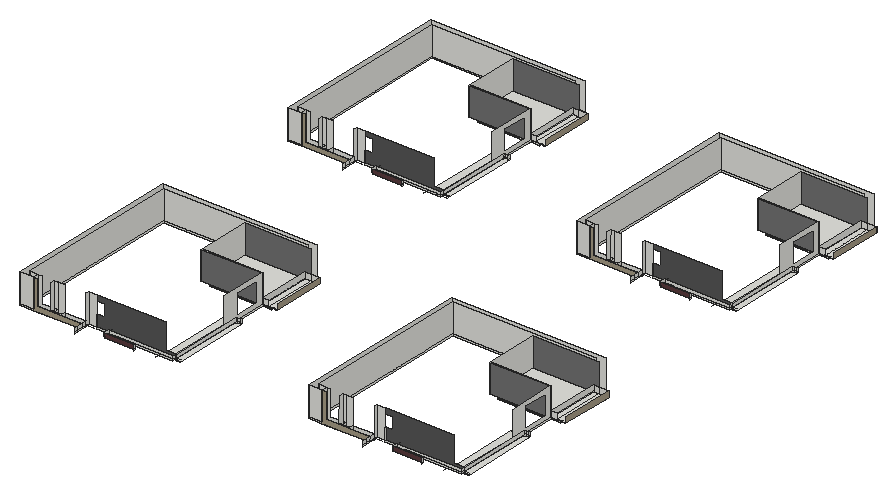
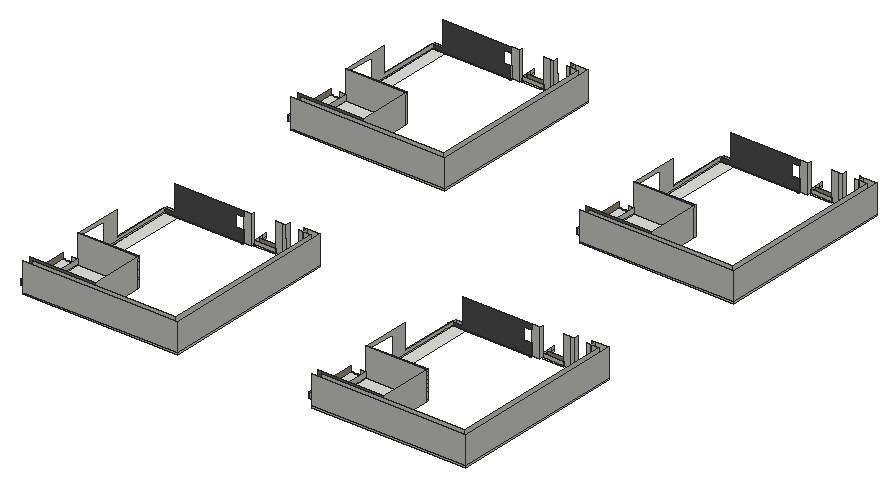
# SketchUp Ruby script. Lengths in inches.
U = 1.inch
M = Sketchup.active_model
def pt(a) = Geom::Point3d.new(a.map { |v| v * U })
def face(e, loops, mat)
  f = e.add_face(loops[0].map { |a| pt(a) })
  loops[1..].each { |l| e.add_face(l.map { |a| pt(a) }).erase! }
  f.material = f.back_material = mat if mat
  f
end
# faces: each face lists its corners as indices into pts; further lists are holes
def faces(e, pts, list, mat = nil) = list.each { |f| face(e, (f[0].is_a?(Array) ? f : [f]).map { |l| l.map { |i| pts[i] } }, mat) }
# xy, xz, yz: faces in a plane at the given z, y or x. An outline is a flat list of corners, or four numbers for a rectangle; further outlines are holes
def ring(l) = l.size == 4 ? [[l[0], l[1]], [l[2], l[1]], [l[2], l[3]], [l[0], l[3]]] : l.each_slice(2).to_a
def flat(e, list, mat, &to3) = list.each { |f| face(e, (f[0].is_a?(Array) ? f : [f]).map { |l| ring(l).map { |u, v| to3.(u, v) } }, mat) }
def xy(e, z, list, mat = nil) = flat(e, list, mat) { |x, y| [x, y, z] }
def xz(e, y, list, mat = nil) = flat(e, list, mat) { |x, z| [x, y, z] }
def yz(e, x, list, mat = nil) = flat(e, list, mat) { |y, z| [x, y, z] }
def lines(e, pts, list) = list.each { |a, b| e.add_line(pt(pts[a]), pt(pts[b])) }
# prism: a flat outline (further loops are holes) pulled along v
def prism(e, loops, v, mat = nil)
  f = face(e, loops, mat); d = Geom::Vector3d.new(v.map { |x| x * U })
  f.pushpull(f.normal.samedirection?(d) ? d.length : -d.length)
end
def box(e, o, s, mat = nil) = prism(e, [[o, [o[0] + s[0], o[1], o[2]], [o[0] + s[0], o[1] + s[1], o[2]], [o[0], o[1] + s[1], o[2]]]], [0, 0, s[2]], mat)
def at(x, y, z, deg = 0) = Geom::Transformation.translation(pt([x, y, z])) * Geom::Transformation.rotation(ORIGIN, Z_AXIS, deg.degrees)
def axes(o, x, y, z) = Geom::Transformation.new([*x, 0, *y, 0, *z, 0, *pt(o).to_a, 1])
def part(name) = M.definitions.add(name)
# library, detail: a bought-in or finely detailed component or shape, given as its bounding box
def library(name, o, s) = part(name).tap { |d| box(d.entities, o, s) }
def detail(e, o, s) = box(e.add_group.entities, o, s)
def put(e, d, t, mat = nil) = e.add_instance(d, t).tap { |i| i.material = mat if mat }
def group(e, t, mat = nil) = e.add_group.tap { |g| g.transformation = t; g.material = mat if mat }.entities
root = M.entities
M.materials.add("[Color M05]").color = [114, 114, 114]
M.materials.add("[Color M06]").color = [86, 86, 86]
M.materials.add("[Concrete Tile]").color = [165, 155, 133]
M.materials.add("[Granite Brown]").color = [89, 59, 61]
xy(root,630,[[319.53,1799.9375,319.53,1822.9375,401.77,1822.9375,401.77,1806.5625,446.15,1806.5625,446.15,1822.9375,523.04,1822.9375,523.04,1799.9375],[1537.72,1799.9375,1537.72,1822.9375,1619.96,1822.9375,1619.96,1806.5625,1664.33,1806.5625,1664.33,1822.9375,1741.23,1822.9375,1741.23,1799.9375],[431.33,1806.5625,446.15,1822.9375],[1649.52,1806.5625,1664.33,1822.9375],[655.61,1822.9375,655.61,1833.5,557.88,1833.5,557.88,1835.1875,890.875,1835.1875,890.875,1822.9375],
  [1873.79,1822.9375,1873.79,1833.5,1776.07,1833.5,1776.07,1835.1875,2109.0625,1835.1875,2109.0625,1822.9375],[838.125,1835.1875,890.875,2148.83],[890.875,1835.1875,890.875,2148.83,894.3125,2148.83,894.3125,2156.01,913.875,2156.01,913.875,1835.1875],[2056.3125,1835.1875,2109.0625,2148.83],[2109.0625,1835.1875,2109.0625,2148.83,2112.5,2148.83,2112.5,2156.01,2132.0625,2156.01,2132.0625,1835.1875],
  [671.875,2290,890.875,2295.875],[1890.0625,2290,2109.0625,2295.875],[671.875,2295.875,890.875,2518.89],[890.875,2295.875,913.875,2518.89],[1890.0625,2295.875,2109.0625,2518.89],
  [2109.0625,2295.875,2132.0625,2518.89],[319.53,3214.625,319.53,3237.625,401.77,3237.625,401.77,3221.25,446.15,3221.25,446.15,3237.625,523.04,3237.625,523.04,3214.625],[1537.72,3214.625,1537.72,3237.625,1619.96,3237.625,1619.96,3221.25,1664.33,3221.25,1664.33,3237.625,1741.23,3237.625,1741.23,3214.625],[431.33,3221.25,446.15,3237.625],[1649.52,3221.25,1664.33,3237.625],
  [655.61,3237.625,655.61,3248.1875,557.88,3248.1875,557.88,3249.875,890.875,3249.875,890.875,3237.625],[1873.79,3237.625,1873.79,3248.1875,1776.07,3248.1875,1776.07,3249.875,2109.0625,3249.875,2109.0625,3237.625],[838.125,3249.875,890.875,3563.51],[890.875,3249.875,890.875,3563.51,894.3125,3563.51,894.3125,3570.7,913.875,3570.7,913.875,3249.875],[2056.3125,3249.875,2109.0625,3563.51],
  [2109.0625,3249.875,2109.0625,3563.51,2112.5,3563.51,2112.5,3570.7,2132.0625,3570.7,2132.0625,3249.875],[671.875,3704.6875,890.875,3710.5625],[1890.0625,3704.6875,2109.0625,3710.5625],[671.875,3710.5625,890.875,3933.57],[890.875,3710.5625,913.875,3933.57],
  [1890.0625,3710.5625,2109.0625,3933.57],[2109.0625,3710.5625,2132.0625,3933.57]])
xy(root,636,[[616.54,1799.9375,618.61,1822.9375],[1834.73,1799.9375,1836.79,1822.9375],[655.61,1822.9375,890.875,1837.0625],[1873.79,1822.9375,2109.0625,1837.0625],[557.88,1833.5,655.61,1833.5,655.61,1837.0625,557.4,1837.0625,557.4,1835.1875,557.88,1835.1875],
  [1776.07,1833.5,1873.79,1833.5,1873.79,1837.0625,1775.59,1837.0625,1775.59,1835.1875,1776.07,1835.1875],[635.3125,2290,890.875,2295.875],[1853.5,2290,2109.0625,2295.875],[635.3125,2295.875,890.875,2518.89],[890.875,2295.875,913.875,2518.89],
  [913.875,2295.875,954.6875,2518.89],[1853.5,2295.875,2109.0625,2518.89],[2109.0625,2295.875,2132.0625,2518.89],[2132.0625,2295.875,2172.875,2518.89],[616.54,3214.625,618.61,3237.625],
  [1834.73,3214.625,1836.79,3237.625],[655.61,3237.625,890.875,3251.75],[1873.79,3237.625,2109.0625,3251.75],[557.88,3248.1875,655.61,3248.1875,655.61,3251.75,557.4,3251.75,557.4,3249.875,557.88,3249.875],[1776.07,3248.1875,1873.79,3248.1875,1873.79,3251.75,1775.59,3251.75,1775.59,3249.875,1776.07,3249.875],
  [635.3125,3704.6875,890.875,3710.5625],[1853.5,3704.6875,2109.0625,3710.5625],[635.3125,3710.5625,890.875,3933.57],[890.875,3710.5625,913.875,3933.57],[913.875,3710.5625,954.6875,3933.57],
  [1853.5,3710.5625,2109.0625,3933.57],[2109.0625,3710.5625,2132.0625,3933.57],[2132.0625,3710.5625,2172.875,3933.57]])
xz(root,1799.9375,[[262.875,630,319.53,636],[1481.0625,630,1537.72,636],[262.875,636,319.53,756],[1481.0625,636,1537.72,756]])
xz(root,1799.9375,[[319.53,630,523.04,630,523.04,651.4375,333.89,651.4375,333.89,756,319.53,756],[1537.72,630,1741.23,630,1741.23,651.4375,1552.08,651.4375,1552.08,756,1537.72,756]],"[Concrete Tile]")
xz(root,1799.9375,[[618.61,630,745.8,630,745.8,648.6875,616.54,648.6875,616.54,636,618.61,636],[1836.79,630,1963.98,630,1963.98,648.6875,1834.73,648.6875,1834.73,636,1836.79,636]],"[Granite Brown]")
xz(root,1806.5625,[[401.8,636,401.8,651.4375,387.07,651.51,386.99,636.07],[401.8,636,401.88,651.4375,401.8,651.4375],[401.8,636,431.33,636,431.33,651.4375,401.88,651.4375],[1619.99,636,1619.99,651.4375,1605.26,651.51,1605.18,636.07],[1619.99,636,1620.07,651.4375,1619.99,651.4375],
  [1619.99,636,1649.52,636,1649.52,651.4375,1620.07,651.4375]])
xz(root,1822.9375,[[618.61,630,655.61,636],[655.61,630,835.99,636],[835.99,630,890.875,636],[1836.79,630,1873.79,636],[1873.79,630,2054.17,636],
  [2054.17,630,2109.0625,636],[285.875,636,319.53,756],[319.53,636,401.8,636,386.99,636.07,387.07,651.4375,333.89,651.4375,333.89,756,319.53,756],[401.8,636,386.99,636.07,387.07,651.4375,401.8,651.4375],[401.8,636,402.4,756,387.59,756,387.07,651.4375,401.8,651.4375],
  [401.8,636,402.4,756,431.33,756,431.33,636],[431.33,636,523.04,651.4375],[616.54,636,890.875,648.6875],[1504.0625,636,1537.72,756],[1537.72,636,1619.99,636,1605.18,636.07,1605.26,651.4375,1552.08,651.4375,1552.08,756,1537.72,756],
  [1619.99,636,1605.18,636.07,1605.26,651.4375,1619.99,651.4375],[1619.99,636,1620.59,756,1605.78,756,1605.26,651.4375,1619.99,651.4375],[1619.99,636,1620.59,756,1649.52,756,1649.52,636],[1649.52,636,1741.23,651.4375],[1834.73,636,2109.0625,648.6875]])
xz(root,1833.5,[[557.88,630,655.61,636],[1776.07,630,1873.79,636]])
xz(root,1835.1875,[[523.04,636,557.4,756],[890.875,636,894.3125,648.6875],[1741.23,636,1775.59,756],[2109.0625,636,2112.5,648.6875]])
xz(root,1835.1875,[[557.4,636,557.88,682.81],[1775.59,636,1776.07,682.81]],"[Granite Brown]")
xz(root,1837.0625,[[[557.4,636,890.875,636,890.875,648.6875,847.6875,648.6875,847.6875,756,557.4,756,557.4,735.09,589.71,735.09,589.71,682.81,557.4,682.81],[611.65,641.5625,632.49,641.875]],[[1775.59,636,2109.0625,636,2109.0625,648.6875,2065.875,648.6875,2065.875,756,1775.59,756,1775.59,735.09,1807.9,735.09,1807.9,682.81,1775.59,682.81],[1829.84,641.5625,1850.67,641.875]]],"[Color M06]")
xz(root,2156.01,[[894.3125,630,913.875,636],[2112.5,630,2132.0625,636],[894.3125,636,913.875,648.6875],[2112.5,636,2132.0625,648.6875]])
xz(root,2290,[[635.3125,636,890.875,756],[1853.5,636,2109.0625,756]],"[Color M05]")
xz(root,2295.875,[[913.875,630,930.75,636],[2132.0625,630,2148.9375,636],[635.3125,636,890.875,756],[890.875,636,913.875,660.0625],[913.875,636,930.75,637.75],
  [930.75,636,954.6875,637.75],[1853.5,636,2109.0625,756],[2109.0625,636,2132.0625,660.0625],[2132.0625,636,2148.9375,637.75],[2148.9375,636,2172.875,637.75]])
xz(root,2518.89,[[890.875,636,913.875,660.0625],[913.875,636,954.6875,660.0625],[2109.0625,636,2132.0625,660.0625],[2132.0625,636,2172.875,660.0625]])
xz(root,2518.89,[[635.3125,636,890.875,636,890.875,660.0625,913.875,660.0625,913.875,756,635.3125,756],[1853.5,636,2109.0625,636,2109.0625,660.0625,2132.0625,660.0625,2132.0625,756,1853.5,756]],"[Color M05]")
xz(root,2531.375,[[285.875,630,890.875,636],[1504.0625,630,2109.0625,636],[285.875,636,890.875,756],[1504.0625,636,2109.0625,756]])
xz(root,2554.375,[[262.875,630,913.875,636],[1481.0625,630,2132.0625,636],[262.875,636,913.875,756],[1481.0625,636,2132.0625,756]])
xz(root,3214.625,[[262.875,630,319.53,636],[1481.0625,630,1537.72,636],[262.875,636,319.53,756],[1481.0625,636,1537.72,756]])
xz(root,3214.625,[[319.53,630,523.04,630,523.04,651.4375,333.89,651.4375,333.89,756,319.53,756],[1537.72,630,1741.23,630,1741.23,651.4375,1552.08,651.4375,1552.08,756,1537.72,756]],"[Concrete Tile]")
xz(root,3214.625,[[618.61,630,745.8,630,745.8,648.6875,616.54,648.6875,616.54,636,618.61,636],[1836.79,630,1963.98,630,1963.98,648.6875,1834.73,648.6875,1834.73,636,1836.79,636]],"[Granite Brown]")
xz(root,3221.25,[[401.8,636,401.8,651.4375,387.07,651.51,386.99,636.07],[401.8,636,401.88,651.4375,401.8,651.4375],[401.8,636,431.33,636,431.33,651.4375,401.88,651.4375],[1619.99,636,1619.99,651.4375,1605.26,651.51,1605.18,636.07],[1619.99,636,1620.07,651.4375,1619.99,651.4375],
  [1619.99,636,1649.52,636,1649.52,651.4375,1620.07,651.4375]])
xz(root,3237.625,[[618.61,630,655.61,636],[655.61,630,835.99,636],[835.99,630,890.875,636],[1836.79,630,1873.79,636],[1873.79,630,2054.17,636],
  [2054.17,630,2109.0625,636],[285.875,636,319.53,756],[319.53,636,401.8,636,386.99,636.07,387.07,651.4375,333.89,651.4375,333.89,756,319.53,756],[401.8,636,386.99,636.07,387.07,651.4375,401.8,651.4375],[401.8,636,402.4,756,387.59,756,387.07,651.4375,401.8,651.4375],
  [401.8,636,402.4,756,431.33,756,431.33,636],[431.33,636,523.04,651.4375],[616.54,636,890.875,648.6875],[1504.0625,636,1537.72,756],[1537.72,636,1619.99,636,1605.18,636.07,1605.26,651.4375,1552.08,651.4375,1552.08,756,1537.72,756],
  [1619.99,636,1605.18,636.07,1605.26,651.4375,1619.99,651.4375],[1619.99,636,1620.59,756,1605.78,756,1605.26,651.4375,1619.99,651.4375],[1619.99,636,1620.59,756,1649.52,756,1649.52,636],[1649.52,636,1741.23,651.4375],[1834.73,636,2109.0625,648.6875]])
xz(root,3248.1875,[[557.88,630,655.61,636],[1776.07,630,1873.79,636]])
xz(root,3249.875,[[523.04,636,557.4,756],[890.875,636,894.3125,648.6875],[1741.23,636,1775.59,756],[2109.0625,636,2112.5,648.6875]])
xz(root,3249.875,[[557.4,636,557.88,682.81],[1775.59,636,1776.07,682.81]],"[Granite Brown]")
xz(root,3251.75,[[[557.4,636,890.875,636,890.875,648.6875,847.6875,648.6875,847.6875,756,557.4,756,557.4,735.09,589.71,735.09,589.71,682.81,557.4,682.81],[611.65,641.5625,632.49,641.875]],[[1775.59,636,2109.0625,636,2109.0625,648.6875,2065.875,648.6875,2065.875,756,1775.59,756,1775.59,735.09,1807.9,735.09,1807.9,682.81,1775.59,682.81],[1829.84,641.5625,1850.67,641.875]]],"[Color M06]")
xz(root,3570.7,[[894.3125,630,913.875,636],[2112.5,630,2132.0625,636],[894.3125,636,913.875,648.6875],[2112.5,636,2132.0625,648.6875]])
xz(root,3704.6875,[[635.3125,636,890.875,756],[1853.5,636,2109.0625,756]],"[Color M05]")
xz(root,3710.5625,[[913.875,630,930.75,636],[2132.0625,630,2148.9375,636],[635.3125,636,890.875,756],[890.875,636,913.875,660.0625],[913.875,636,930.75,637.75],
  [930.75,636,954.6875,637.75],[1853.5,636,2109.0625,756],[2109.0625,636,2132.0625,660.0625],[2132.0625,636,2148.9375,637.75],[2148.9375,636,2172.875,637.75]])
xz(root,3933.57,[[890.875,636,913.875,660.0625],[913.875,636,954.6875,660.0625],[2109.0625,636,2132.0625,660.0625],[2132.0625,636,2172.875,660.0625]])
xz(root,3933.57,[[635.3125,636,890.875,636,890.875,660.0625,913.875,660.0625,913.875,756,635.3125,756],[1853.5,636,2109.0625,636,2109.0625,660.0625,2132.0625,660.0625,2132.0625,756,1853.5,756]],"[Color M05]")
xz(root,3946.0625,[[285.875,630,890.875,636],[1504.0625,630,2109.0625,636],[285.875,636,890.875,756],[1504.0625,636,2109.0625,756]])
xz(root,3969.0625,[[262.875,630,913.875,636],[1481.0625,630,2132.0625,636],[262.875,636,913.875,756],[1481.0625,636,2132.0625,756]])
yz(root,262.875,[[1799.9375,630,2554.375,636],[3214.625,630,3969.0625,636],[1799.9375,636,2554.375,756],[3214.625,636,3969.0625,756]])
yz(root,285.875,[[1822.9375,630,2531.375,636],[3237.625,630,3946.0625,636],[1822.9375,636,2531.375,756],[3237.625,636,3946.0625,756]])
yz(root,319.53,[[1799.9375,636,1822.9375,756],[3214.625,636,3237.625,756]])
yz(root,401.8,[[1806.5625,636,1822.9375,651.4375],[3221.25,636,3237.625,651.4375]])
yz(root,431.33,[[1806.5625,636,1822.9375,651.4375],[3221.25,636,3237.625,651.4375]])
yz(root,523.04,[[1763.25,630,1799.9375,636],[3177.9375,630,3214.625,636],[1763.25,636,1799.9375,651.4375],[1799.9375,636,1822.9375,651.4375],[1822.9375,636,1835.1875,756],
  [3177.9375,636,3214.625,651.4375],[3214.625,636,3237.625,651.4375],[3237.625,636,3249.875,756]])
yz(root,557.4,[[1835.1875,636,1837.0625,682.81],[3249.875,636,3251.75,682.81]])
yz(root,616.54,[[1799.9375,636,1822.9375,648.6875],[3214.625,636,3237.625,648.6875]])
yz(root,618.61,[[1799.9375,630,1822.9375,636],[3214.625,630,3237.625,636]])
yz(root,635.3125,[[2290,636,2295.875,756],[2295.875,636,2518.89,756],[3704.6875,636,3710.5625,756],[3710.5625,636,3933.57,756]])
yz(root,655.61,[[1822.9375,630,1833.5,636],[3237.625,630,3248.1875,636]])
yz(root,745.8,[[1795.6875,630,1799.9375,636],[3210.375,630,3214.625,636],[1795.6875,636,1799.9375,648.6875],[3210.375,636,3214.625,648.6875]])
yz(root,890.875,[[1822.9375,630,1835.1875,636],[1835.1875,630,2531.375,636],[3237.625,630,3249.875,636],[3249.875,630,3946.0625,636],[1822.9375,636,1835.1875,648.6875],
  [1835.1875,636,1837.0625,648.6875],[[1837.0625,636,1837.0625,648.6875,2091.0625,648.6875,2091.0625,756,2290,756,2290,636],[2156.01,653.36,2266.33,739.04]],[2290,636,2295.875,637.75],[2295.875,636,2518.89,660.0625],[3237.625,636,3249.875,648.6875],
  [3249.875,636,3251.75,648.6875],[[3251.75,636,3251.75,648.6875,3505.75,648.6875,3505.75,756,3704.6875,756,3704.6875,636],[3570.7,653.36,3681.01,739.04]],[3704.6875,636,3710.5625,637.75],[3710.5625,636,3933.57,660.0625]])
yz(root,894.3125,[[2148.83,630,2156.01,636],[3563.51,630,3570.7,636],[1835.1875,636,2148.83,648.6875],[2148.83,636,2156.01,648.6875],[3249.875,636,3563.51,648.6875],
  [3563.51,636,3570.7,648.6875]])
yz(root,913.875,[[2148.83,630,2156.01,636],[3563.51,630,3570.7,636],[2148.83,636,2156.01,648.6875],[3563.51,636,3570.7,648.6875]])
yz(root,954.6875,[[2295.875,636,2518.89,660.0625],[3710.5625,636,3933.57,660.0625]],"[Concrete Tile]")
yz(root,1481.0625,[[1799.9375,630,2554.375,636],[3214.625,630,3969.0625,636],[1799.9375,636,2554.375,756],[3214.625,636,3969.0625,756]])
yz(root,1504.0625,[[1822.9375,630,2531.375,636],[3237.625,630,3946.0625,636],[1822.9375,636,2531.375,756],[3237.625,636,3946.0625,756]])
yz(root,1537.72,[[1799.9375,636,1822.9375,756],[3214.625,636,3237.625,756]])
yz(root,1619.99,[[1806.5625,636,1822.9375,651.4375],[3221.25,636,3237.625,651.4375]])
yz(root,1649.52,[[1806.5625,636,1822.9375,651.4375],[3221.25,636,3237.625,651.4375]])
yz(root,1741.23,[[1763.25,630,1799.9375,636],[3177.9375,630,3214.625,636],[1763.25,636,1799.9375,651.4375],[1799.9375,636,1822.9375,651.4375],[1822.9375,636,1835.1875,756],
  [3177.9375,636,3214.625,651.4375],[3214.625,636,3237.625,651.4375],[3237.625,636,3249.875,756]])
yz(root,1775.59,[[1835.1875,636,1837.0625,682.81],[3249.875,636,3251.75,682.81]])
yz(root,1834.73,[[1799.9375,636,1822.9375,648.6875],[3214.625,636,3237.625,648.6875]])
yz(root,1836.79,[[1799.9375,630,1822.9375,636],[3214.625,630,3237.625,636]])
yz(root,1853.5,[[2290,636,2295.875,756],[2295.875,636,2518.89,756],[3704.6875,636,3710.5625,756],[3710.5625,636,3933.57,756]])
yz(root,1873.79,[[1822.9375,630,1833.5,636],[3237.625,630,3248.1875,636]])
yz(root,1963.98,[[1795.6875,630,1799.9375,636],[3210.375,630,3214.625,636],[1795.6875,636,1799.9375,648.6875],[3210.375,636,3214.625,648.6875]])
yz(root,2109.0625,[[1822.9375,630,1835.1875,636],[1835.1875,630,2531.375,636],[3237.625,630,3249.875,636],[3249.875,630,3946.0625,636],[1822.9375,636,1835.1875,648.6875],
  [1835.1875,636,1837.0625,648.6875],[[1837.0625,636,1837.0625,648.6875,2091.0625,648.6875,2091.0625,756,2290,756,2290,636],[2156.01,653.36,2266.33,739.04]],[2290,636,2295.875,637.75],[2295.875,636,2518.89,660.0625],[3237.625,636,3249.875,648.6875],
  [3249.875,636,3251.75,648.6875],[[3251.75,636,3251.75,648.6875,3505.75,648.6875,3505.75,756,3704.6875,756,3704.6875,636],[3570.7,653.36,3681.01,739.04]],[3704.6875,636,3710.5625,637.75],[3710.5625,636,3933.57,660.0625]])
yz(root,2112.5,[[2148.83,630,2156.01,636],[3563.51,630,3570.7,636],[1835.1875,636,2148.83,648.6875],[2148.83,636,2156.01,648.6875],[3249.875,636,3563.51,648.6875],
  [3563.51,636,3570.7,648.6875]])
yz(root,2132.0625,[[2148.83,630,2156.01,636],[3563.51,630,3570.7,636],[2148.83,636,2156.01,648.6875],[3563.51,636,3570.7,648.6875]])
yz(root,2172.875,[[2295.875,636,2518.89,660.0625],[3710.5625,636,3933.57,660.0625]],"[Concrete Tile]")
p = [[401.8,1822.9375,636],[401.8,1806.5625,636],[386.99,1806.5625,636.07],[386.99,1822.9375,636.07],[1619.99,1822.9375,636],[1619.99,1806.5625,636],
  [1605.18,1806.5625,636.07],[1605.18,1822.9375,636.07],[401.8,3237.625,636],[401.8,3221.25,636],[386.99,3221.25,636.07],[386.99,3237.625,636.07],
  [1619.99,3237.625,636],[1619.99,3221.25,636],[1605.18,3221.25,636.07],[1605.18,3237.625,636.07],[387.07,1806.5625,651.51],[387.59,1806.5625,756.07],
  [387.59,1822.9375,756.07],[387.59,1822.9375,756],[387.07,1822.9375,651.4375],[1605.26,1806.5625,651.51],[1605.78,1806.5625,756.07],[1605.78,1822.9375,756.07],
  [1605.78,1822.9375,756],[1605.26,1822.9375,651.4375],[387.07,3221.25,651.51],[387.59,3221.25,756.07],[387.59,3237.625,756.07],[387.59,3237.625,756],
  [387.07,3237.625,651.4375],[1605.26,3221.25,651.51],[1605.78,3221.25,756.07],[1605.78,3237.625,756.07],[1605.78,3237.625,756],[1605.26,3237.625,651.4375],
  [1741.23,1822.9375,636],[1775.59,1822.9375,636],[2132.0625,1827.4375,630],[2112.5,1827.4375,630],[2112.5,1835.1875,630],[2054.17,1822.9375,636],
  [2054.17,1795.6875,636],[2112.5,1835.1875,636],[2132.0625,1835.1875,636],[1741.23,1778.3125,636],[1741.23,1778.3125,651.4375],[1741.23,1778.3125,630],
  [523.04,1822.9375,636],[557.4,1822.9375,636],[913.875,1827.4375,630],[894.3125,1827.4375,630],[894.3125,1835.1875,630],[835.99,1822.9375,636],
  [835.99,1795.6875,636],[894.3125,1835.1875,636],[913.875,1835.1875,636],[523.04,1778.3125,636],[523.04,1778.3125,651.4375],[523.04,1778.3125,630],
  [1741.23,3237.625,636],[1775.59,3237.625,636],[1741.23,3193,636],[1741.23,3193,651.4375],[1741.23,3193,630],[2132.0625,3242.125,630],
  [2112.5,3242.125,630],[2112.5,3249.875,630],[2054.17,3237.625,636],[2054.17,3210.375,636],[2112.5,3249.875,636],[2132.0625,3249.875,636],
  [913.875,3242.125,630],[894.3125,3242.125,630],[894.3125,3249.875,630],[894.3125,3249.875,636],[913.875,3249.875,636],[835.99,3237.625,636],
  [835.99,3210.375,636],[523.04,3237.625,636],[557.4,3237.625,636],[523.04,3193,636],[523.04,3193,651.4375],[523.04,3193,630]]
faces(root,p,[[0,1,2,3],[4,5,6,7],[8,9,10,11],[12,13,14,15],[3,2,16,17,18,19,20],[7,6,21,22,23,24,25],[11,10,26,27,28,29,30],[15,14,31,32,33,34,35]])
lines(root,p,[[36,37],[38,39],[39,40],[41,42],[43,44],[45,46],[47,45],[48,49],[50,51],[51,52],[53,54],[55,56],
  [57,58],[59,57],[60,61],[62,63],[64,62],[65,66],[66,67],[68,69],[70,71],[72,73],[73,74],[75,76],
  [77,78],[79,80],[81,82],[83,81]])
